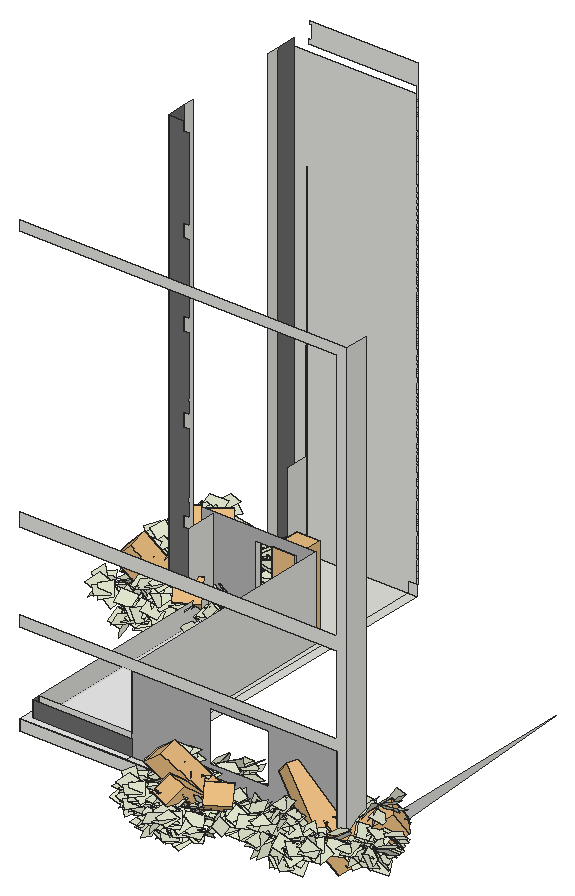
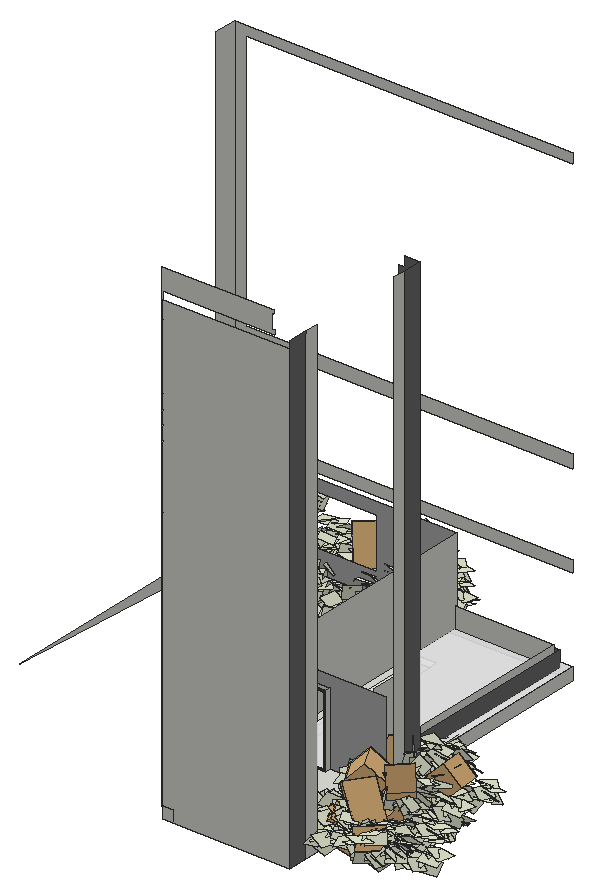
# SketchUp Ruby script. Lengths in inches.
U = 1.inch
M = Sketchup.active_model
def pt(a) = Geom::Point3d.new(a.map { |v| v * U })
def face(e, loops, mat)
  f = e.add_face(loops[0].map { |a| pt(a) })
  loops[1..].each { |l| e.add_face(l.map { |a| pt(a) }).erase! }
  f.material = f.back_material = mat if mat
  f
end
# faces: each face lists its corners as indices into pts; further lists are holes
def faces(e, pts, list, mat = nil) = list.each { |f| face(e, (f[0].is_a?(Array) ? f : [f]).map { |l| l.map { |i| pts[i] } }, mat) }
# xy, xz, yz: faces in a plane at the given z, y or x. An outline is a flat list of corners, or four numbers for a rectangle; further outlines are holes
def ring(l) = l.size == 4 ? [[l[0], l[1]], [l[2], l[1]], [l[2], l[3]], [l[0], l[3]]] : l.each_slice(2).to_a
def flat(e, list, mat, &to3) = list.each { |f| face(e, (f[0].is_a?(Array) ? f : [f]).map { |l| ring(l).map { |u, v| to3.(u, v) } }, mat) }
def xy(e, z, list, mat = nil) = flat(e, list, mat) { |x, y| [x, y, z] }
def xz(e, y, list, mat = nil) = flat(e, list, mat) { |x, z| [x, y, z] }
def yz(e, x, list, mat = nil) = flat(e, list, mat) { |y, z| [x, y, z] }
def lines(e, pts, list) = list.each { |a, b| e.add_line(pt(pts[a]), pt(pts[b])) }
# prism: a flat outline (further loops are holes) pulled along v
def prism(e, loops, v, mat = nil)
  f = face(e, loops, mat); d = Geom::Vector3d.new(v.map { |x| x * U })
  f.pushpull(f.normal.samedirection?(d) ? d.length : -d.length)
end
def box(e, o, s, mat = nil) = prism(e, [[o, [o[0] + s[0], o[1], o[2]], [o[0] + s[0], o[1] + s[1], o[2]], [o[0], o[1] + s[1], o[2]]]], [0, 0, s[2]], mat)
def at(x, y, z, deg = 0) = Geom::Transformation.translation(pt([x, y, z])) * Geom::Transformation.rotation(ORIGIN, Z_AXIS, deg.degrees)
def axes(o, x, y, z) = Geom::Transformation.new([*x, 0, *y, 0, *z, 0, *pt(o).to_a, 1])
def part(name) = M.definitions.add(name)
# library, detail: a bought-in or finely detailed component or shape, given as its bounding box
def library(name, o, s) = part(name).tap { |d| box(d.entities, o, s) }
def detail(e, o, s) = box(e.add_group.entities, o, s)
def put(e, d, t, mat = nil) = e.add_instance(d, t).tap { |i| i.material = mat if mat }
def group(e, t, mat = nil) = e.add_group.tap { |g| g.transformation = t; g.material = mat if mat }.entities
root = M.entities
M.materials.add("Celtis_australis_s cópia1").color = [224, 229, 205]
M.materials.add("Niraj_Hair_Dark").color = [109, 109, 109]
M.materials.add("Niraj_Hair_Gray").color = [178, 178, 178]
M.materials.add("Tendaggio").color = [239, 239, 239]
M.materials["Tendaggio"].alpha = 0.9
M.materials.add("[Asphalt New]").color = [67, 60, 62]
c1 = part("leaf1\#1")
p = [[1.6,6.78,0.04],[-9.34,-4.04,0.02],[2.67,-16.2,2.05],[13.62,-5.38,2.07]]
faces(c1.entities,p,[[0,1,2,3]],"Celtis_australis_s cópia1")
c2 = part("leaf_group1\#1")
put(c2.entities,c1,axes([-0.06,3.68,7.3125],[0.53029,-0.80282,-0.27253],[0.82812,0.42159,0.36943],[-0.18168,-0.42159,0.8884]))
put(c2.entities,c1,axes([6.4375,-3.58,5.23],[1,0,0],[0,0.98927,0.14608],[0,-0.14608,0.98927]))
put(c2.entities,c1,axes([-0.99,3.68,1.22],[0.57591,-0.80282,0.15431],[0.36532,0.42159,0.82994],[-0.73135,-0.42159,0.53609]))
put(c2.entities,c1,axes([18.71,8.59,4.39],[0.33053,0.77491,0.53877],[-0.79988,-0.073,0.5957],[0.50094,-0.62785,0.5957]))
put(c2.entities,c1,axes([13.16,0.76,0.89],[0.89618,0.3501,0.27256],[-0.44248,0.65988,0.60727],[0.03275,-0.66482,0.74628]))
put(c2.entities,c1,axes([4.53,7.98,7.3125],[-0.1927,0.94265,-0.27253],[0.88368,0.28746,0.36943],[-0.42658,0.16964,0.8884]))
put(c2.entities,c1,axes([12.46,21.28,7.16],[0.85019,0.38493,0.35918],[0.30538,-0.91629,0.25914],[-0.42887,0.11063,0.89657]))
put(c2.entities,c1,axes([6.53,15.18,2.59],[0.70711,0.70711,0],[0.5,-0.5,0.70711],[-0.5,0.5,0.70711]))
put(c2.entities,c1,axes([-3.17,8.15,3.46],[-0.03719,0.74973,0.66069],[0.94096,-0.19634,0.27576],[-0.33647,-0.63194,0.69817]))
put(c2.entities,c1,axes([23.03,17.79,4.39],[0.78166,-0.31422,0.53877],[-0.61722,-0.51398,0.5957],[-0.08973,0.79818,0.5957]))
put(c2.entities,c1,axes([14.78,21.52,3.21],[0.67246,-0.04394,0.73882],[-0.28657,-0.93583,0.20517],[-0.6824,0.3497,0.64191]))
put(c2.entities,c1,axes([10.37,-1.8125,9],[0.99279,-0.06448,-0.101],[0.11527,0.74421,0.65792],[0.03275,-0.66482,0.74628]))
put(c2.entities,c1,axes([1.45,16.1875,2.9375],[-0.2106,-0.86579,-0.45394],[0.96054,-0.26957,0.06852],[-0.18168,-0.42159,0.8884]))
c3 = library("branch1\#2",[0,0,0],[33.4,33.29,108.01])
c4 = library("Tenda",[0,0,0],[9.09,66.93,111.26])
xy(root,109.91,[[494.79,89.375,494.79,301.21,500.29,301.21,500.29,464.11,597.61,464.11,595.48,143.4375,595.48,134.5,834.53,134.5,834.53,89.375],[595.48,143.4375,597.61,464.11,607.36,464.11,605.23,143.4375],[479.54,301.21,500.29,354.38],[479.54,354.38,500.29,464.11]])
xy(root,121.74,[[605.23,89.375,823.9,96.6875],[597.61,153,605.23,336.16]])
xy(root,121.74,[[494.79,89.375,605.23,89.375,605.23,96.6875,502.29,96.6875,502.29,319.0625,505.92,319.0625,505.92,99.4375,605.23,99.4375,605.23,153,597.61,153,597.61,336.16,580.61,336.16,580.61,341.53,541.86,341.53,541.86,336.16,500.29,336.16,500.29,301.21,494.79,301.21]],"Tendaggio")
xz(root,89.375,[[494.79,109.91,834.53,109.91,834.53,585.8125,494.79,585.8125,494.79,575.91,823.9,575.91,823.9,314.1875,494.79,314.1875,494.79,300.47,823.9,300.47,823.9,218.5625,494.79,218.5625,494.79,207.01,823.9,207.01,823.9,121.74,494.79,121.74]])
xz(root,96.6875,[[502.29,121.74,605.23,138.27]],"Niraj_Hair_Dark")
xz(root,96.6875,[[[605.23,121.74,823.9,207.01],[686.21,143.64,747.21,195.52]]],"Niraj_Hair_Gray")
xz(root,99.4375,[[505.92,121.74,605.23,142.68]])
xz(root,301.21,[[494.79,109.91,500.29,121.74]])
xz(root,301.21,[[479.54,109.91,494.79,109.91,494.79,121.74,500.29,121.74,500.29,207.01,494.79,207.01,494.79,218.5625,500.29,218.5625,500.29,231.41,499.48,231.41,499.48,235.75,500.29,235.75,500.29,300.47,494.79,300.47,494.79,314.1875,500.29,314.1875,500.29,325.23,499.98,325.23,499.98,328.3125,500.29,328.3125,500.29,389.4,494.79,389.4,494.79,403.5,500.29,403.5,500.29,476.89,494.79,476.89,494.79,490.8125,500.29,490.8125,500.29,575.91,494.79,575.91,494.79,585.8125,479.54,585.8125]],"Niraj_Hair_Dark")
xz(root,319.0625,[[502.29,121.74,505.92,142.68]])
xz(root,336.16,[[500.29,121.74,541.86,121.74,541.86,195.13,580.61,195.13,580.61,121.74,605.23,121.74,605.23,207.01,485.73,207.01,485.73,125.43,500.29,125.43]],"Niraj_Hair_Gray")
xz(root,341.53,[[[541.86,121.74,580.61,195.13],[543.67,123.55,578.8,193.32]]],"[Asphalt New]")
xz(root,464.11,[[479.54,109.91,479.54,578.41,607.36,578.41,607.36,121.74,597.61,121.74,597.61,109.91],[597.61,109.91,607.36,121.74],[607.36,121.74,607.36,585.8125,495.23,585.8125,495.23,590.04,497.79,590.04,497.79,604.78,495.92,604.78,495.92,607.875,608.47,607.875,608.47,121.74]])
yz(root,479.54,[[321.37,109.91,321.37,585.8125,333.01,585.8125,333.01,125.43,430.89,125.43,430.89,585.8125,443.75,585.8125,443.75,109.91]])
yz(root,479.54,[[301.21,109.91,321.37,585.8125],[443.75,109.91,464.11,585.8125]],"Niraj_Hair_Dark")
yz(root,494.79,[[89.375,109.91,301.21,121.74]])
yz(root,500.29,[[301.21,109.91,301.21,121.74,336.16,121.74,336.16,125.43,354.38,125.43,354.38,109.91],[354.38,109.91,454.49,109.91,454.49,310.625,454.11,310.625,454.11,224.0625,454.18,224.0625,454.18,207.01,430.89,207.01,430.89,125.43,354.38,125.43],[454.49,109.91,455.3,476.89],[301.21,121.74,333.01,207.01],[333.01,121.74,336.16,125.43]])
yz(root,502.29,[[96.6875,121.74,96.6875,138.27,311.625,138.27,311.625,142.68,319.0625,142.68,319.0625,121.74]],"Niraj_Hair_Dark")
yz(root,505.92,[[99.4375,121.74,319.0625,142.68]])
yz(root,541.86,[[336.16,121.74,341.53,195.13]])
yz(root,580.61,[[336.16,121.74,341.53,195.13]],"[Asphalt New]")
yz(root,605.23,[[99.4375,121.74,99.4375,142.68,96.6875,142.68,96.6875,207.01,336.16,207.01,336.16,121.74]])
yz(root,823.9,[[89.375,121.74,96.6875,207.01]])
yz(root,834.53,[[89.375,109.91,134.5,109.91,360.375,124.25,113.9375,124.25,113.9375,585.8125,89.375,585.8125]])
put(root,c2,axes([645.34,47.05,111.91],[0.59429,0.64993,-0.09956],[-0.65681,0.60058,0],[0.0867,0.09481,0.68247]))
put(root,c2,axes([693.27,121.84,112.18],[0.03841,0.87984,-0.09956],[-0.88915,0.03882,0],[0.0056,0.12835,0.68247]))
put(root,c2,axes([733.63,116.4375,112.22],[-0.03841,-0.87984,-0.09956],[0.88915,-0.03882,0],[-0.0056,-0.12835,0.68247]))
put(root,c2,axes([804.11,131.35,116.3125],[-0.03841,-0.87984,-0.12848],[0.88915,-0.03882,0],[-0.0056,-0.12835,0.88068]))
put(root,c2,axes([819.02,112.1,116.3125],[-0.03841,-0.87984,-0.12848],[0.88915,-0.03882,0],[-0.0056,-0.12835,0.88068]))
put(root,c2,axes([460.71,377.71,112.23],[-0.04316,-0.98858,-0.09672],[0.99905,-0.04362,0],[-0.0063,-0.14422,0.66298]))
put(root,c2,axes([427.97,335.56,116.7],[0.7444,0.47059,-0.12848],[-0.47557,0.75228,0],[0.1086,0.06865,0.88068]))
put(root,c2,axes([496.86,382.75,112.4],[-0.04316,-0.98858,-0.09672],[0.99905,-0.04362,0],[-0.0063,-0.14422,0.66298]))
put(root,c2,axes([648.91,80.73,110.06],[0.58229,-0.67221,-0.02648],[0.67271,0.58272,0],[0.02237,-0.02582,0.68919]))
put(root,c2,axes([443.34,338.96,112.86],[0.59551,-0.79027,-0.09672],[0.79864,0.60182,0],[0.08688,-0.11529,0.66298]))
put(root,c3,axes([462.98,405.46,99.65],[0.36963,-0.70636,0.04462],[-0.51774,-0.21719,0.38183],[0.28265,0.17853,0.21763]))
put(root,c2,axes([669.91,94.85,113.54],[0.53001,-0.70334,-0.09956],[0.71079,0.53562,0],[0.07732,-0.10261,0.68247]))
put(root,c4,axes([560.13,334.76,100],[0,3.55421,0],[0.35907,0,0],[0,0,0.87048]))
put(root,c2,axes([445,303.75,122.54],[0.53001,-0.68244,-0.21324],[0.71079,0.53162,0.06528],[0.07732,-0.20917,0.86161]))
put(root,c2,axes([395.19,394.5625,113.4375],[0.59551,-0.79027,-0.09672],[0.79864,0.60182,0],[0.08688,-0.11529,0.66298]))
put(root,c2,axes([466.55,262.27,123.62],[0.74921,0.45418,0.15655],[-0.41604,0.75843,-0.20928],[-0.24021,0.10299,0.85076]))
put(root,c3,axes([485.58,333.59,100.41],[-0.57341,-0.41789,0.05927],[-0.259,0.42733,0.50721],[0.24895,-0.28903,0.37063]))
put(root,c2,axes([495.24,374.28,113.71],[0.04316,0.98858,-0.09672],[-0.99905,0.04362,0],[0.0063,0.14422,0.66298]))
put(root,c3,axes([836.14,77.16,100.48],[-0.49147,0.51069,0.06785],[-0.24614,-0.31515,0.5891],[0.40731,0.34486,0.35468]))
put(root,c2,axes([764.28,66.16,114.24],[0.58229,-0.67221,-0.03417],[0.67271,0.58272,0],[0.02237,-0.02582,0.88934]))
put(root,c2,axes([506.98,398.44,113.95],[-0.83641,0.52876,-0.09672],[-0.53435,-0.84526,0],[-0.12202,0.07714,0.66298]))
put(root,c2,axes([447.13,344.76,124.18],[0.74921,0.45418,0.15655],[-0.41604,0.75843,-0.20928],[-0.24021,0.10299,0.85076]))
put(root,c2,axes([726.86,123.73,121.09],[0.0391,-0.87984,-0.0994],[0.74059,-0.03882,0.38131],[-0.49203,-0.12835,0.56604]))
put(root,c2,axes([414.45,380.5,114.93],[0.59576,-0.79027,-0.09602],[0.79863,0.60182,0.00093],[0.08515,-0.11529,0.66308]))
put(root,c2,axes([678.36,31.36,119.18],[0.53001,-0.68244,-0.16524],[0.71079,0.53162,0.05058],[0.07732,-0.20917,0.6677]))
put(root,c2,axes([713.08,23.64,119.18],[0.26509,0.82241,-0.16524],[-0.83972,0.2876,0.05058],[0.12922,0.18175,0.6677]))
put(root,c2,axes([743.78,94.83,115.54],[-0.04763,0.87939,-0.09956],[-0.8887,-0.04813,0],[-0.00695,0.12829,0.68247]))
put(root,c2,axes([654.4,94.87,115.74],[0.53001,-0.70334,-0.09956],[0.71079,0.53562,0],[0.07732,-0.10261,0.68247]))
put(root,c2,axes([478.94,314.08,115.59],[-0.46214,0.87795,0.08376],[-0.88678,-0.45652,-0.04836],[-0.0063,-0.14422,0.66298]))
put(root,c2,axes([428.6,416.82,118.18],[-0.04897,-0.98032,0.12812],[0.95241,0.01183,0.20407],[-0.30086,0.19704,0.62517]))
put(root,c2,axes([680.49,92.95,121.28],[0.74921,0.45418,0.12132],[-0.41604,0.75843,-0.16218],[-0.24021,0.10299,0.65929]))
put(root,c2,axes([430.92,334.15,149.52],[0.33028,-0.70334,-0.43397],[0.5516,0.53562,-0.44828],[0.61543,-0.10261,0.63468]))
put(root,c2,axes([700.55,23,117.29],[0.88068,0,-0.09956],[0,0.89,0],[0.12848,0,0.68247]))
put(root,c2,axes([483.84,331.54,116.92],[0.59756,0.78872,-0.09672],[-0.79707,0.60388,0],[0.08717,0.11506,0.66298]))
put(root,c2,axes([415.4,335.56,121.71],[0.7444,0.47059,-0.12848],[-0.47557,0.75228,0],[0.1086,0.06865,0.88068]))
put(root,c2,axes([492.6,317.1875,121.84],[-0.03841,-0.87984,-0.12848],[0.88915,-0.03882,0],[-0.0056,-0.12835,0.88068]))
put(root,c2,axes([433.67,401.01,118.13],[0.04229,0.99083,0.08597],[-0.96813,0.00891,0.16769],[0.24685,-0.13481,0.64295]))
put(root,c2,axes([459.03,334.05,122.08],[0.84181,0.51031,0.11785],[-0.46746,0.85217,-0.15755],[-0.2699,0.11572,0.64046]))
put(root,c2,axes([631.18,66.63,119.28],[0.55423,-0.68442,-0.09956],[0.69166,0.5601,0],[0.08085,-0.09985,0.68247]))
put(root,c2,axes([646.48,42.29,119.28],[0.88068,0,-0.09956],[0,0.89,0],[0.12848,0,0.68247]))
put(root,c2,axes([859.54,102.28,123.32],[-0.04763,0.87939,-0.12848],[-0.8887,-0.04813,0],[-0.00695,0.12829,0.88068]))
put(root,c2,axes([850.47,102.28,123.32],[-0.04763,0.87939,-0.12848],[-0.8887,-0.04813,0],[-0.00695,0.12829,0.88068]))
put(root,c3,axes([460.81,406.69,105.89],[-0.5941,-0.51953,0.02355],[0.35927,-0.37036,0.4008],[-0.29023,0.35871,0.26558]))
put(root,c2,axes([445,301.39,129.46],[0.53001,-0.69763,0.15655],[0.71079,0.49304,-0.20928],[0.07732,0.24966,0.85076]))
put(root,c2,axes([517.54,318.2,123.73],[0.03841,0.87984,-0.12848],[-0.88915,0.03882,0],[0.0056,0.12835,0.88068]))
put(root,c2,axes([678.36,29,124.55],[0.53001,-0.69763,0.12132],[0.71079,0.49304,-0.16218],[0.07732,0.24966,0.65929]))
put(root,c3,axes([455.97,319.4,106.7],[-0.12279,0.69882,0.05927],[0.49771,0.04443,0.50721],[-0.36911,-0.09629,0.37063]))
put(root,c2,axes([683.96,139.8,120.67],[-0.03841,-0.87984,-0.09956],[0.88915,-0.03882,0],[-0.0056,-0.12835,0.68247]))
put(root,c2,axes([467.19,274.8125,125.27],[0.88068,0,-0.12848],[0,0.89,0],[0.12848,0,0.88068]))
put(root,c2,axes([413.125,294.1,125.27],[0.88068,0,-0.12848],[0,0.89,0],[0.12848,0,0.88068]))
put(root,c2,axes([877.35,80.09,126.1],[-0.59498,0.6493,-0.12848],[-0.65618,-0.60128,0],[-0.0868,0.09472,0.88068]))
put(root,c3,axes([709.08,65.52,108.63],[-0.66136,0.25698,0.04593],[0.21982,0.44874,0.39305],[-0.10884,-0.3656,0.28722]))
put(root,c2,axes([421.68,429.5625,143.48],[0.3711,-0.79027,-0.32669],[0.61978,0.60182,-0.33747],[0.69149,-0.11529,0.4778]))
put(root,c2,axes([804.11,120.83,126.32],[-0.03841,-0.87984,-0.12848],[0.88915,-0.03882,0],[-0.0056,-0.12835,0.88068]))
put(root,c2,axes([499.34,390.29,122.03],[0.59756,0.78872,-0.09672],[-0.79707,0.60388,0],[0.08717,0.11506,0.66298]))
put(root,c2,axes([743.78,63.18,123.125],[-0.04763,0.87939,-0.09956],[-0.8887,-0.04813,0],[-0.00695,0.12829,0.68247]))
put(root,c2,axes([732.05,48.96,123.125],[0.75804,0.4483,-0.09956],[-0.45305,0.76606,0],[0.11059,0.0654,0.68247]))
put(root,c2,axes([417.47,428.88,124.97],[-0.04897,-0.98032,0.12812],[0.95241,0.01183,0.20407],[-0.30086,0.19704,0.62517]))
put(root,c2,axes([733.63,123.73,123.9],[-0.03841,-0.87984,-0.09956],[0.88915,-0.03882,0],[-0.0056,-0.12835,0.68247]))
put(root,c2,axes([438.25,361.64,123.7],[-0.98953,0,-0.09672],[0,-1,0],[-0.14436,0,0.66298]))
put(root,c2,axes([406.4375,364.25,123.7],[0.98953,0,-0.09672],[0,1,0],[0.14436,0,0.66298]))
put(root,c2,axes([468.8,432.88,123.83],[-0.04316,-0.98858,-0.09672],[0.99905,-0.04362,0],[-0.0063,-0.14422,0.66298]))
put(root,c2,axes([829.05,121.84,128.22],[0.03841,0.87984,-0.12848],[-0.88915,0.03882,0],[0.0056,0.12835,0.88068]))
put(root,c2,axes([460.25,401.08,123.29],[-0.46214,0.87795,0.08376],[-0.88678,-0.45652,-0.04836],[-0.0063,-0.14422,0.66298]))
put(root,c2,axes([646.48,47.01,124.92],[0.88068,0,-0.09956],[0,0.89,0],[0.12848,0,0.68247]))
put(root,c2,axes([424.32,330.6,124.64],[0.98943,0.01382,-0.09672],[-0.01396,0.9999,0],[0.14434,0.00202,0.66298]))
put(root,c3,axes([466.18,368.68,111.48],[-0.7431,0.28874,0.04462],[0.24699,0.5042,0.38183],[-0.09539,-0.32042,0.21763]))
put(root,c2,axes([468.04,331.66,129.74],[-0.03841,-0.87984,-0.12848],[0.88915,-0.03882,0],[-0.0056,-0.12835,0.88068]))
put(root,c2,axes([500.22,336.15,129.96],[-0.03841,-0.87984,-0.12848],[0.88915,-0.03882,0],[-0.0056,-0.12835,0.88068]))
put(root,c2,axes([661.33,83.74,126.13],[0.7444,0.47059,-0.09956],[-0.47557,0.75228,0],[0.1086,0.06865,0.68247]))
put(root,c2,axes([452.59,297.18,130.57],[0.53001,-0.70334,-0.12848],[0.71079,0.53562,0],[0.07732,-0.10261,0.88068]))
put(root,c3,axes([470.07,356.36,113.03],[0.32897,-0.62866,0.05927],[-0.46078,-0.1933,0.50721],[0.25156,0.15889,0.28909]))
put(root,c2,axes([678.36,51.9375,130.65],[0.53001,-0.68244,-0.16524],[0.71079,0.53162,0.05058],[0.07732,-0.20917,0.6677]))
put(root,c2,axes([699.91,10.46,131.49],[0.74921,0.45418,0.12132],[-0.41604,0.75843,-0.16218],[-0.24021,0.10299,0.65929]))
put(root,c3,axes([718.94,81.78,113.51],[-0.57341,-0.41789,0.04593],[-0.259,0.42733,0.39305],[0.24895,-0.28903,0.28722]))
put(root,c2,axes([828.72,31.51,130.56],[-0.41131,0.78137,0.11126],[-0.78924,-0.4063,-0.06424],[-0.0056,-0.12835,0.88068]))
put(root,c2,axes([409.73,346.67,131.33],[0.53001,-0.70334,-0.12848],[0.71079,0.53562,0],[0.07732,-0.10261,0.88068]))
put(root,c2,axes([680.49,92.95,131.92],[0.74921,0.45418,0.12132],[-0.41604,0.75843,-0.16218],[-0.24021,0.10299,0.65929]))
put(root,c2,axes([469.54,402.7,127.17],[0.97051,-0.19308,-0.09672],[0.19512,0.98078,0],[0.14158,-0.02817,0.66298]))
put(root,c2,axes([469.54,335.01,127.17],[0.97051,-0.19308,-0.09672],[0.19512,0.98078,0],[0.14158,-0.02817,0.66298]))
put(root,c2,axes([498.78,328.62,131.7],[0.03841,0.87984,-0.12848],[-0.88915,0.03882,0],[0.0056,0.12835,0.88068]))
put(root,c2,axes([509.22,350.12,132.02],[-0.7444,0.47059,-0.12848],[-0.47557,-0.75228,0],[-0.1086,0.06865,0.88068]))
put(root,c3,axes([815.27,101.53,116.45],[-0.27649,-0.65344,-0.05927],[0.44202,-0.23304,0.50721],[-0.4364,0.14415,0.44654]))
put(root,c2,axes([852.4,80.54,132.33],[0.59498,-0.6493,-0.12848],[0.65618,0.60128,0],[0.0868,-0.09472,0.88068]))
put(root,c2,axes([445.21,339.1,133.22],[0.98039,-0.08879,0.11785],[0.12944,0.9633,-0.15755],[-0.14857,0.25331,0.64046]))
put(root,c2,axes([426.87,334.15,133.3125],[0.53023,-0.70334,-0.12755],[0.71078,0.53562,0.00124],[0.07578,-0.10261,0.88081]))
put(root,c2,axes([664.28,82.34,151.56],[0.33028,-0.70334,-0.3363],[0.5516,0.53562,-0.34739],[0.61543,-0.10261,0.49184]))
put(root,c2,axes([820.7,57.43,133.375],[0.88068,0,-0.12848],[0,0.89,0],[0.12848,0,0.88068]))
put(root,c2,axes([648.76,83.74,130.01],[0.7444,0.47059,-0.09956],[-0.47557,0.75228,0],[0.1086,0.06865,0.68247]))
put(root,c2,axes([765.49,47.05,134.04],[0.59429,0.64993,-0.12848],[-0.65681,0.60058,0],[0.0867,0.09481,0.88068]))
put(root,c2,axes([725.96,65.375,130.11],[-0.03841,-0.87984,-0.09956],[0.88915,-0.03882,0],[-0.0056,-0.12835,0.68247]))
put(root,c2,axes([481.83,413.82,129.89],[-0.04316,-0.98858,-0.09672],[0.99905,-0.04362,0],[-0.0063,-0.14422,0.66298]))
put(root,c2,axes([813.42,121.84,134.39],[0.03841,0.87984,-0.12848],[-0.88915,0.03882,0],[0.0056,0.12835,0.88068]))
put(root,c2,axes([853.78,116.4375,134.45],[-0.03841,-0.87984,-0.12848],[0.88915,-0.03882,0],[-0.0056,-0.12835,0.88068]))
put(root,c2,axes([484.27,275.03,134.19],[-0.41131,0.78137,0.11126],[-0.78924,-0.4063,-0.06424],[-0.0056,-0.12835,0.88068]))
put(root,c2,axes([439.47,366.47,137.64],[-0.04359,-0.87249,0.17019],[0.84765,0.01053,0.27108],[-0.26776,0.17537,0.83045]))
put(root,c2,axes([406.4375,372.4375,130.9],[0.98953,0,-0.09672],[0,1,0],[0.14436,0,0.66298]))
put(root,c2,axes([479.09,378.6,130.95],[0.59756,0.78872,-0.09672],[-0.79707,0.60388,0],[0.08717,0.11506,0.66298]))
put(root,c3,axes([457.78,410.15,130.41],[-0.5154,-0.60822,0.04462],[0.39602,-0.39798,-0.38183],[0.27176,-0.19472,0.21763]))
put(root,c2,axes([480.66,392.59,131.02],[-0.47101,-0.87024,-0.09672],[0.87945,-0.47599,0],[-0.06871,-0.12695,0.66298]))
put(root,c2,axes([678.36,49.58,136.02],[0.53001,-0.69763,0.12132],[0.71079,0.49304,-0.16218],[0.07732,0.24966,0.65929]))
put(root,c2,axes([750.9,66.39,131.58],[0.03841,0.87984,-0.09956],[-0.88915,0.03882,0],[0.0056,0.12835,0.68247]))
put(root,c2,axes([769.06,80.73,131.66],[0.58229,-0.67221,-0.03417],[0.67271,0.58272,0],[0.02237,-0.02582,0.88934]))
put(root,c2,axes([488.63,290.58,135.97],[0.53183,0.70196,-0.12848],[-0.70939,0.53746,0],[0.07759,0.10241,0.88068]))
put(root,c3,axes([689.33,67.59,118.375],[-0.12279,0.69882,0.04593],[0.49771,0.04443,0.39305],[-0.36911,-0.09629,0.28722]))
put(root,c2,axes([790.06,94.85,136.15],[0.53001,-0.70334,-0.12848],[0.71079,0.53562,0],[0.07732,-0.10261,0.88068]))
put(root,c2,axes([437.82,414.58,131.42],[-0.46214,0.87795,0.08376],[-0.88678,-0.45652,-0.04836],[-0.0063,-0.14422,0.66298]))
put(root,c2,axes([437.82,401.08,131.42],[-0.46214,0.87795,0.08376],[-0.88678,-0.45652,-0.04836],[-0.0063,-0.14422,0.66298]))
put(root,c2,axes([700.55,23,132.77],[0.88068,0,-0.09956],[0,0.89,0],[0.12848,0,0.68247]))
put(root,c2,axes([646.48,42.29,132.77],[0.88068,0,-0.09956],[0,0.89,0],[0.12848,0,0.68247]))
put(root,c2,axes([443.98,352.41,137.57],[0.03764,0.88184,0.1142],[-0.86164,0.00793,0.22275],[0.21969,-0.11998,0.85407]))
put(root,c2,axes([432.57,351.5,132.57],[0.59551,-0.79027,-0.09672],[0.79864,0.60182,0],[0.08688,-0.11529,0.66298]))
put(root,c2,axes([466.55,292.81,142.8125],[0.74921,0.45418,0.15655],[-0.41604,0.75843,-0.20928],[-0.24021,0.10299,0.85076]))
put(root,c2,axes([847.01,123.73,145.89],[0.0391,-0.87984,-0.12827],[0.74059,-0.03882,0.49205],[-0.49203,-0.12835,0.73043]))
put(root,c2,axes([833.23,23.64,143.43],[0.26509,0.82241,-0.21324],[-0.83972,0.2876,0.06528],[0.12922,0.18175,0.86161]))
put(root,c2,axes([798.51,31.36,143.43],[0.53001,-0.68244,-0.21324],[0.71079,0.53162,0.06528],[0.07732,-0.20917,0.86161]))
put(root,c2,axes([863.93,94.83,138.73],[-0.04763,0.87939,-0.12848],[-0.8887,-0.04813,0],[-0.00695,0.12829,0.88068]))
put(root,c3,axes([468.13,357.46,121.31],[-0.52875,-0.46238,0.03129],[0.31975,-0.32962,0.53241],[-0.2583,0.31925,0.35278]))
put(root,c2,axes([774.55,94.87,138.99],[0.53001,-0.70334,-0.12848],[0.71079,0.53562,0],[0.07732,-0.10261,0.88068]))
